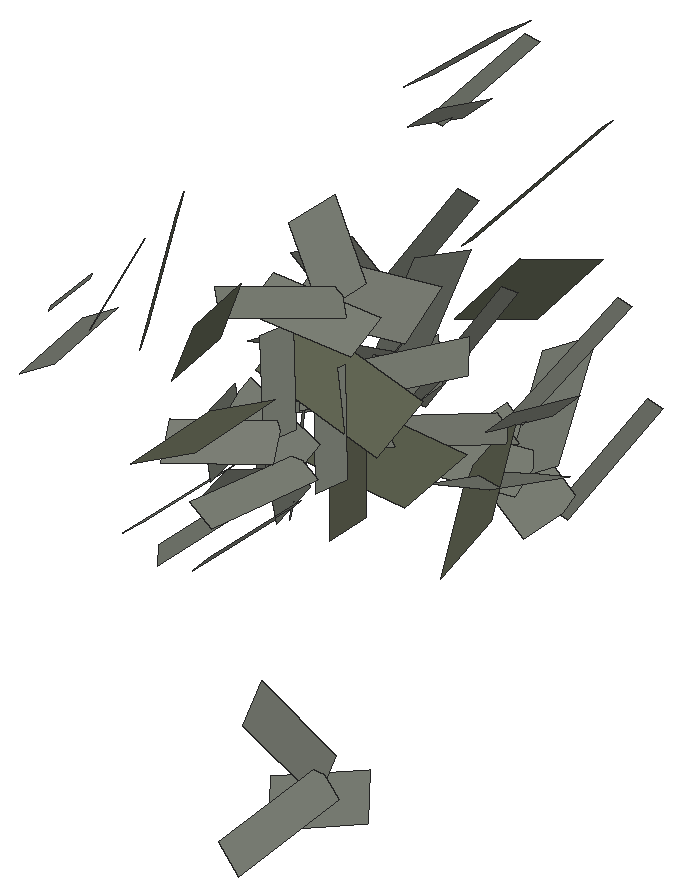
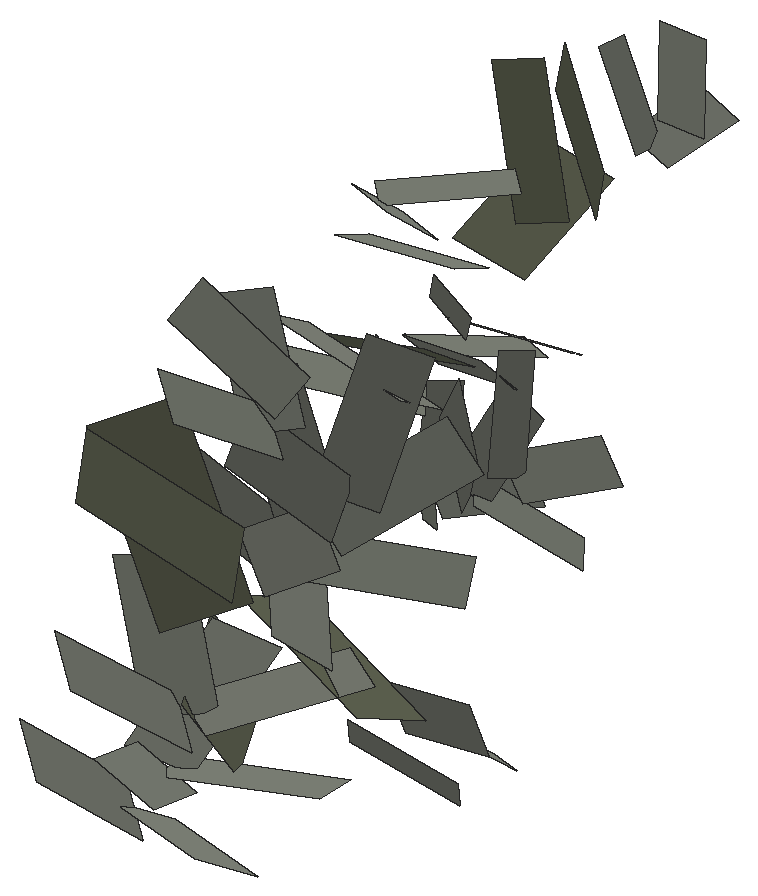
# SketchUp Ruby script. Lengths in inches.
U = 1.inch
M = Sketchup.active_model
def pt(a) = Geom::Point3d.new(a.map { |v| v * U })
def face(e, loops, mat)
  f = e.add_face(loops[0].map { |a| pt(a) })
  loops[1..].each { |l| e.add_face(l.map { |a| pt(a) }).erase! }
  f.material = f.back_material = mat if mat
  f
end
# faces: each face lists its corners as indices into pts; further lists are holes
def faces(e, pts, list, mat = nil) = list.each { |f| face(e, (f[0].is_a?(Array) ? f : [f]).map { |l| l.map { |i| pts[i] } }, mat) }
# xy, xz, yz: faces in a plane at the given z, y or x. An outline is a flat list of corners, or four numbers for a rectangle; further outlines are holes
def ring(l) = l.size == 4 ? [[l[0], l[1]], [l[2], l[1]], [l[2], l[3]], [l[0], l[3]]] : l.each_slice(2).to_a
def flat(e, list, mat, &to3) = list.each { |f| face(e, (f[0].is_a?(Array) ? f : [f]).map { |l| ring(l).map { |u, v| to3.(u, v) } }, mat) }
def xy(e, z, list, mat = nil) = flat(e, list, mat) { |x, y| [x, y, z] }
def xz(e, y, list, mat = nil) = flat(e, list, mat) { |x, z| [x, y, z] }
def yz(e, x, list, mat = nil) = flat(e, list, mat) { |y, z| [x, y, z] }
def lines(e, pts, list) = list.each { |a, b| e.add_line(pt(pts[a]), pt(pts[b])) }
# prism: a flat outline (further loops are holes) pulled along v
def prism(e, loops, v, mat = nil)
  f = face(e, loops, mat); d = Geom::Vector3d.new(v.map { |x| x * U })
  f.pushpull(f.normal.samedirection?(d) ? d.length : -d.length)
end
def box(e, o, s, mat = nil) = prism(e, [[o, [o[0] + s[0], o[1], o[2]], [o[0] + s[0], o[1] + s[1], o[2]], [o[0], o[1] + s[1], o[2]]]], [0, 0, s[2]], mat)
def at(x, y, z, deg = 0) = Geom::Transformation.translation(pt([x, y, z])) * Geom::Transformation.rotation(ORIGIN, Z_AXIS, deg.degrees)
def axes(o, x, y, z) = Geom::Transformation.new([*x, 0, *y, 0, *z, 0, *pt(o).to_a, 1])
def part(name) = M.definitions.add(name)
# library, detail: a bought-in or finely detailed component or shape, given as its bounding box
def library(name, o, s) = part(name).tap { |d| box(d.entities, o, s) }
def detail(e, o, s) = box(e.add_group.entities, o, s)
def put(e, d, t, mat = nil) = e.add_instance(d, t).tap { |i| i.material = mat if mat }
def group(e, t, mat = nil) = e.add_group.tap { |g| g.transformation = t; g.material = mat if mat }.entities
root = M.entities
M.materials.add("viburnumblaasdfas0df1w06d").color = [98, 102, 84]
M.materials.add("viburnumbladsadfasdfad0w122").color = [125, 129, 119]
c1 = part("Component\#315")
p = [[0.25,0,0],[2.05,0.01,0.35],[1.81,4.2,1.66],[0,4.19,1.3125]]
faces(c1.entities,p,[[0,1,2,3]],"viburnumbladsadfasdfad0w122")
c2 = part("viburnumblad2")
put(c2.entities,c1,axes([-19.23,-4.49,-32.18],[83.35428,0,0],[0,79.38502,0],[0,0,83.35428]))
c3 = part("Component\#314")
p = [[0.14,0,0],[2.58,0.05,0.25],[2.44,5.11,2.64],[0,5.05,2.39]]
faces(c3.entities,p,[[0,1,2,3]],"viburnumblaasdfas0df1w06d")
c4 = part("viburnumblad1\#2")
put(c4.entities,c3,axes([-37.25,6.23,19.31],[75.98784,0,0],[0,65.50676,0],[0,0,75.98784]))
put(root,c2,axes([1217.99,269.35,20.33],[-0.0062,0.00344,-0.00762],[-0.00004,-0.00961,-0.00424],[-0.0081,-0.00223,0.0048]))
put(root,c2,axes([1215.85,281.99,26.62],[0.01052,-0.00734,0.00272],[0.00582,0.00933,0.00265],[-0.0036,-0.00095,0.01134]))
put(root,c2,axes([1216.76,263.93,29.11],[-0.0036,-0.00676,-0.00701],[0.00718,-0.00608,0.00197],[-0.00593,-0.00439,0.00637]))
put(root,c2,axes([1219.82,275.97,20.31],[-0.00427,0.01006,-0.00619],[-0.01054,-0.00775,-0.00533],[-0.00749,0.00313,0.01026]))
put(root,c2,axes([1218.93,269.28,19.32],[-0.00506,0.00898,-0.002],[-0.00471,-0.00455,-0.00828],[-0.00753,-0.00286,0.00529]))
put(root,c2,axes([1217.82,263.85,28.28],[-0.00729,-0.00007,-0.00611],[0.00282,-0.00961,-0.00317],[-0.00621,-0.00405,0.00634]))
put(root,c2,axes([1215.875,282.32,28.0625],[0.00228,-0.01232,0.00076],[0.0106,0.00221,0.00397],[-0.00422,0.00003,0.01117]))
put(root,c2,axes([1219.18,276.68,21.77],[-0.00935,0.0021,-0.00891],[-0.00409,-0.01235,0.00138],[-0.00819,0.00377,0.00948]))
put(root,c2,axes([1220.17,280.75,15.21],[-0.00305,0.01398,0.00068],[-0.01364,-0.00282,-0.0033],[-0.00279,-0.00128,0.01326]))
put(root,c2,axes([1218.14,277.67,22.87],[-0.00877,-0.00751,-0.00615],[0.00336,-0.01013,0.00757],[-0.0091,0.00349,0.00872]))
put(root,c2,axes([1217.44,270.55,20.27],[0.00095,-0.00927,-0.00479],[0.00517,-0.00382,0.00808],[-0.00874,-0.00294,0.00329]))
put(root,c4,axes([1221.02,275.27,17.1],[0.00387,0.01311,0.00437],[-0.0121,0.00667,-0.00928],[-0.00906,-0.00102,0.01108]))
put(root,c2,axes([1217.14,282.08,27.03],[-0.00587,-0.00963,-0.00252],[0.00967,-0.00694,0.00401],[-0.00471,0.00005,0.01098]))
put(root,c2,axes([1220.28,280.85,17.1],[-0.01149,0.00801,-0.00297],[-0.00766,-0.01186,-0.00235],[-0.00352,-0.00017,0.01315]))
put(root,c2,axes([1218.64,276.375,19.21],[0.00916,0.00784,0.00642],[-0.00492,0.00961,-0.00471],[-0.00802,0.00094,0.01029]))
put(root,c2,axes([1217.57,277.09,20.17],[0.00935,-0.0021,0.00891],[0.00182,0.01184,0.00088],[-0.00893,0.00067,0.00953]))
put(root,c2,axes([1217,264.62,28.18],[0.0036,-0.00945,-0.00418],[0.00709,-0.00011,0.00601],[-0.00594,-0.00519,0.00581]))
put(root,c2,axes([1217.04,278.21,21.75],[0.00445,-0.01048,0.00645],[0.00766,0.00772,0.00727],[-0.00963,0.0013,0.00876]))
put(root,c4,axes([1217.81,265.92,26.23],[0.00672,-0.00928,0.00091],[0.00601,0.00561,0.01016],[-0.00772,-0.00461,0.00599]))
put(root,c2,axes([1220.09,281.29,13.46],[0.00689,0.01128,0.00378],[-0.0129,0.00838,-0.00151],[-0.003,-0.00258,0.01303]))
put(root,c2,axes([1218.1,270.91,19.05],[0.00506,-0.00898,0.002],[0.00284,0.00386,0.00969],[-0.00844,-0.00386,0.00315]))
put(root,c2,axes([1219.04,270.8,18.125],[0.00595,-0.0033,0.00732],[-0.00208,0.00949,0.0057],[-0.00787,-0.00449,0.00364]))
put(root,c2,axes([1218.82,270.6,19.99],[-0.00371,-0.00412,-0.00878],[0.00371,-0.00856,0.0023],[-0.0086,-0.00227,0.00398]))
put(root,c4,axes([1217.16,282.58,21.68],[0.00673,-0.01108,0.00456],[0.01197,0.00933,0.00501],[-0.00603,0.0015,0.01157]))
put(root,c2,axes([1218.95,281.77,14.89],[0.0132,0.00264,0.00489],[-0.00375,0.01436,0.00234],[-0.00402,-0.00331,0.01259]))
put(root,c2,axes([1219.97,270.18,19.41],[-0.00487,0.00336,-0.00745],[-0.00004,-0.00961,-0.00424],[-0.00872,-0.00185,0.00395]))
put(root,c2,axes([1221.41,267.1,22.56],[-0.00345,0.00905,0.004],[-0.00954,-0.00184,-0.00399],[-0.00252,-0.00485,0.0079]))
put(root,c2,axes([1218.79,278.15,21.0625],[-0.00306,-0.01272,0.00021],[0.00831,-0.00183,0.01011],[-0.0097,0.00247,0.00842]))
put(root,c2,axes([1222.02,272.75,24.8],[0.00095,0.01366,0.00535],[-0.01286,0.00336,-0.00628],[-0.00706,-0.00428,0.01216]))
put(root,c2,axes([1221.35,267.95,21.51],[0.00404,0.00727,0.00631],[-0.0093,0.00487,0.00025],[-0.00255,-0.00567,0.00738]))
put(root,c2,axes([1219.54,271.22,19.27],[0.00099,-0.00968,-0.005],[0.00466,-0.00344,0.00728],[-0.00874,-0.00294,0.00329]))
put(root,c2,axes([1218.48,282.62,16.7],[0.01149,-0.00801,0.00297],[0.00658,0.01147,0.00547],[-0.00527,-0.00304,0.01219]))
put(root,c2,axes([1220.39,267.94,22.61],[0.00916,0.00124,0.00492],[-0.00387,0.00837,0.00487],[-0.00322,-0.0061,0.00681]))
put(root,c2,axes([1219.03,277.72,19.375],[0.00502,-0.00971,0.00503],[0.00766,0.00772,0.00727],[-0.00909,0.00016,0.0094]))
put(root,c2,axes([1221.75,268.76,9.95],[0.00409,0.00375,0.00971],[-0.00938,0.00585,0.00169],[-0.00452,-0.00876,0.00528]))
put(root,c4,axes([1219.48,267.07,25.78],[-0.00104,-0.01037,-0.00489],[0.01073,-0.00422,0.00645],[-0.0067,-0.00317,0.00766]))
put(root,c4,axes([1221.875,275.8,14.625],[0.00862,0.00382,0.01082],[-0.00301,0.01604,-0.00327],[-0.01117,-0.00026,0.009]))
put(root,c2,axes([1221.43,269.53,27.0625],[0.00759,0.00699,0.00431],[-0.00767,0.00813,0.00032],[-0.00293,-0.00317,0.01031]))
put(root,c2,axes([1221.3,282.09,15.76],[-0.0132,-0.00264,-0.00489],[0.00251,-0.01421,0.00089],[-0.00477,0.0001,0.01275]))
put(root,c2,axes([1222.66,269.48,25.94],[0.00024,0.01092,0.00238],[-0.01143,0.00081,-0.00255],[-0.00254,-0.00227,0.01065]))
put(root,c4,axes([1219.29,282.59,19.66],[-0.0079,-0.01248,0.00117],[0.01398,-0.00821,0.00596],[-0.0035,0.004,0.01323]))
put(root,c2,axes([1222.73,269.17,27.47],[-0.00725,0.00846,-0.00094],[-0.008,-0.0072,-0.00303],[-0.00289,-0.00129,0.01072]))
put(root,c4,axes([1221.25,272.27,17.83],[0.00244,-0.01122,0.00057],[0.00459,0.00184,0.0121],[-0.01018,-0.00173,0.00319]))
put(root,c4,axes([1223.68,270.39,22.01],[0.00232,0.01057,0.00577],[-0.01348,0.00407,-0.00203],[-0.00316,-0.00514,0.01068]))
put(root,c2,axes([1222.58,267.93,22.06],[-0.00892,0.00552,-0.00065],[-0.0045,-0.00791,-0.00542],[-0.00314,-0.00411,0.00807]))
put(root,c4,axes([1221.51,267.25,24.46],[-0.01085,-0.00246,-0.00558],[0.00478,-0.01321,-0.00344],[-0.00438,-0.00417,0.00964]))
put(root,c2,axes([1220.1875,282.65,17.29],[-0.00718,-0.01175,-0.00394],[0.01087,-0.00815,0.00451],[-0.0058,-0.00063,0.01231]))
put(root,c2,axes([1221.58,269.02,20.78],[0.0088,0.00119,0.00472],[-0.00418,0.00904,0.00526],[-0.00322,-0.0061,0.00681]))
put(root,c2,axes([1219.83,283.09,13.64],[0.012,-0.00837,0.00311],[0.00592,0.01032,0.00492],[-0.00527,-0.00304,0.01219]))
put(root,c2,axes([1222.95,268.32,10.55],[-0.00876,0.00688,0.00103],[-0.00474,-0.00469,-0.00897],[-0.00509,-0.00746,0.00659]))
put(root,c2,axes([1223.27,269.34,9.38],[-0.0033,0.00751,0.0076],[-0.0089,0.00112,-0.00498],[-0.00448,-0.00819,0.00616]))
put(root,c2,axes([1223.96,273.45,24.04],[-0.00774,0.01238,-0.00167],[-0.01057,-0.00772,-0.00819],[-0.0074,-0.00296,0.01235]))
